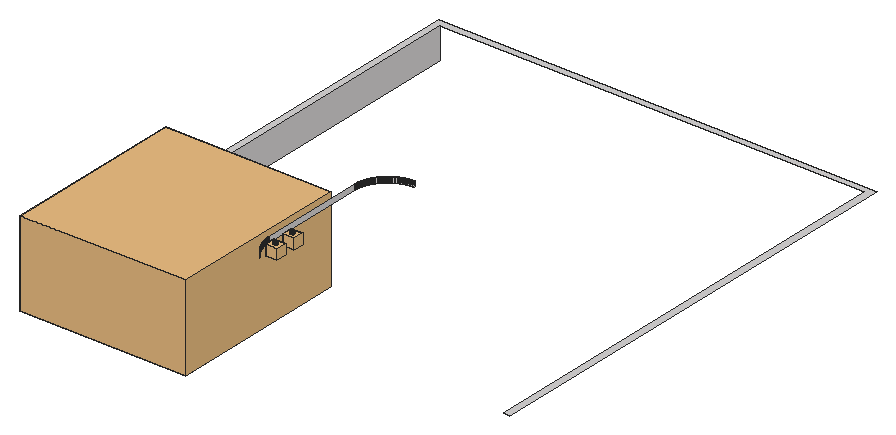
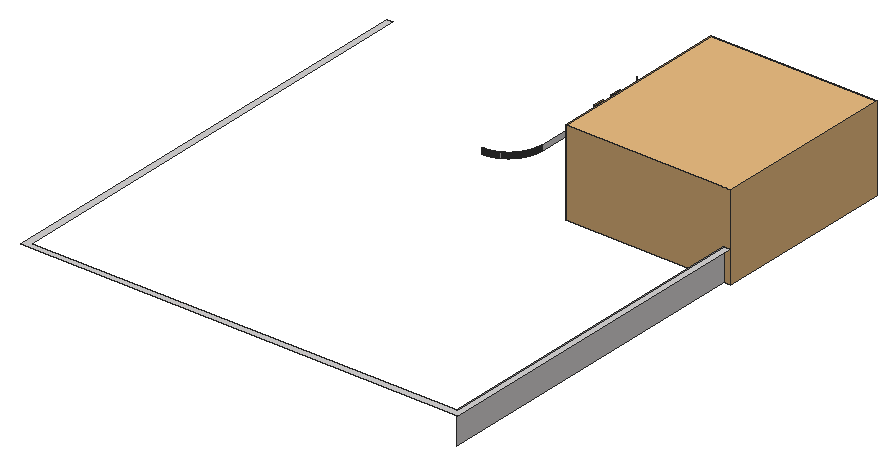
# SketchUp Ruby script. Lengths in inches.
U = 1.inch
M = Sketchup.active_model
def pt(a) = Geom::Point3d.new(a.map { |v| v * U })
def face(e, loops, mat)
  f = e.add_face(loops[0].map { |a| pt(a) })
  loops[1..].each { |l| e.add_face(l.map { |a| pt(a) }).erase! }
  f.material = f.back_material = mat if mat
  f
end
# faces: each face lists its corners as indices into pts; further lists are holes
def faces(e, pts, list, mat = nil) = list.each { |f| face(e, (f[0].is_a?(Array) ? f : [f]).map { |l| l.map { |i| pts[i] } }, mat) }
# xy, xz, yz: faces in a plane at the given z, y or x. An outline is a flat list of corners, or four numbers for a rectangle; further outlines are holes
def ring(l) = l.size == 4 ? [[l[0], l[1]], [l[2], l[1]], [l[2], l[3]], [l[0], l[3]]] : l.each_slice(2).to_a
def flat(e, list, mat, &to3) = list.each { |f| face(e, (f[0].is_a?(Array) ? f : [f]).map { |l| ring(l).map { |u, v| to3.(u, v) } }, mat) }
def xy(e, z, list, mat = nil) = flat(e, list, mat) { |x, y| [x, y, z] }
def xz(e, y, list, mat = nil) = flat(e, list, mat) { |x, z| [x, y, z] }
def yz(e, x, list, mat = nil) = flat(e, list, mat) { |y, z| [x, y, z] }
def lines(e, pts, list) = list.each { |a, b| e.add_line(pt(pts[a]), pt(pts[b])) }
# prism: a flat outline (further loops are holes) pulled along v
def prism(e, loops, v, mat = nil)
  f = face(e, loops, mat); d = Geom::Vector3d.new(v.map { |x| x * U })
  f.pushpull(f.normal.samedirection?(d) ? d.length : -d.length)
end
def box(e, o, s, mat = nil) = prism(e, [[o, [o[0] + s[0], o[1], o[2]], [o[0] + s[0], o[1] + s[1], o[2]], [o[0], o[1] + s[1], o[2]]]], [0, 0, s[2]], mat)
def at(x, y, z, deg = 0) = Geom::Transformation.translation(pt([x, y, z])) * Geom::Transformation.rotation(ORIGIN, Z_AXIS, deg.degrees)
def axes(o, x, y, z) = Geom::Transformation.new([*x, 0, *y, 0, *z, 0, *pt(o).to_a, 1])
def part(name) = M.definitions.add(name)
# library, detail: a bought-in or finely detailed component or shape, given as its bounding box
def library(name, o, s) = part(name).tap { |d| box(d.entities, o, s) }
def detail(e, o, s) = box(e.add_group.entities, o, s)
def put(e, d, t, mat = nil) = e.add_instance(d, t).tap { |i| i.material = mat if mat }
def group(e, t, mat = nil) = e.add_group.tap { |g| g.transformation = t; g.material = mat if mat }.entities
root = M.entities
M.materials.add("[Quartz Light Brown]").color = [215, 212, 212]
M.materials.add("[Wood Veneer 01]").color = [93, 57, 34]
c1 = library("Group\#53",[0,0,-93.56],[180,199,93.56])
c2 = library("3",[-5.26,-4.28,-11.86],[13.52,11.56,11.86])
xy(root,432,[[0,276.5,7,276.5,7,787,488,787,488,276.5,495,276.5,495,794,0,794]],"[Quartz Light Brown]")
xy(root,483,[[193.9375,318.7,193.78,318.71,193.47,318.77,193.32,318.82,193.18,318.88,193.04,318.95,192.9,319.03,192.77,319.12,192.65,319.22,192.54,319.33,192.44,319.45,192.26,319.71,192.19,319.85,192.13,319.99,192.08,320.14,192.04,320.29,192,320.61,192,320.76,192.01,320.92,192.04,321.08,192.07,321.23,192.12,321.38,192.18,321.52,192.25,321.66,192.33,321.8,192.42,321.93,192.52,322.05,192.63,322.16,192.75,322.26,192.875,322.35,193.01,322.4375,193.15,322.51,193.29,322.57,193.44,322.62,193.59,322.66,193.75,322.69,193.91,322.7,194.0625,322.7,194.22,322.6875,194.375,322.67,194.53,322.63,194.68,322.58,194.82,322.52,194.96,322.45,195.1,322.37,195.23,322.28,195.35,322.18,195.46,322.07,195.56,321.95,195.65,321.83,195.74,321.69,195.81,321.55,195.87,321.41,195.92,321.26,195.96,321.11,195.98,320.95,196,320.8,196,320.64,195.99,320.48,195.96,320.33,195.93,320.17,195.88,320.02,195.82,319.88,195.75,319.74,195.67,319.6,195.58,319.48,195.48,319.36,195.37,319.24,195.25,319.14,195.125,319.05,194.99,318.96,194.85,318.89,194.71,318.83,194.56,318.78,194.41,318.74,194.09,318.7],[193.9375,342.7,193.78,342.71,193.47,342.77,193.32,342.82,193.18,342.88,193.04,342.95,192.9,343.03,192.77,343.12,192.65,343.22,192.54,343.33,192.44,343.45,192.26,343.71,192.19,343.85,192.13,343.99,192.08,344.14,192.04,344.29,192,344.61,192,344.76,192.01,344.92,192.04,345.08,192.07,345.23,192.12,345.38,192.18,345.52,192.25,345.66,192.33,345.8,192.42,345.93,192.52,346.05,192.63,346.16,192.75,346.26,192.875,346.35,193.01,346.4375,193.15,346.51,193.29,346.57,193.44,346.62,193.59,346.66,193.75,346.69,193.91,346.7,194.0625,346.7,194.22,346.6875,194.375,346.67,194.53,346.63,194.68,346.58,194.82,346.52,194.96,346.45,195.1,346.37,195.23,346.28,195.35,346.18,195.46,346.07,195.56,345.95,195.65,345.83,195.74,345.69,195.81,345.55,195.87,345.41,195.92,345.26,195.96,345.11,195.98,344.95,196,344.8,196,344.64,195.99,344.48,195.96,344.33,195.93,344.17,195.88,344.02,195.82,343.88,195.75,343.74,195.67,343.6,195.58,343.48,195.48,343.36,195.37,343.24,195.25,343.14,195.125,343.05,194.99,342.96,194.85,342.89,194.71,342.83,194.56,342.78,194.41,342.74,194.09,342.7]],"[Quartz Light Brown]")
xz(root,318.7,[[193.9375,480,194.09,483]],"[Quartz Light Brown]")
xz(root,322.7,[[193.91,480,194.0625,483]],"[Quartz Light Brown]")
xz(root,342.7,[[193.9375,480,194.09,483]],"[Quartz Light Brown]")
xz(root,346.7,[[193.91,480,194.0625,483]],"[Quartz Light Brown]")
xz(root,478.7,[[224.5,480,225,486]],"[Quartz Light Brown]")
yz(root,7,[[276.5,396,787,432]],"[Quartz Light Brown]")
yz(root,187,[[320.2,480,320.7,486],[320.7,480,440.7,486],[440.7,480,441.2,486]],"[Quartz Light Brown]")
yz(root,192,[[320.61,480,320.76,483],[344.61,480,344.76,483]],"[Quartz Light Brown]")
yz(root,196,[[320.64,480,320.8,483],[344.64,480,344.8,483]],"[Quartz Light Brown]")
p = [[198.13,293.83,480],[198.48,293.48,480],[198.48,293.48,486],[198.13,293.83,486],[197.78,294.18,480],[197.78,294.18,486],
  [197.4375,294.54,480],[197.4375,294.54,486],[197.1,294.91,480],[197.1,294.91,486],[196.76,295.27,480],[196.76,295.27,486],
  [196.43,295.65,480],[196.43,295.65,486],[196.1,296.02,480],[196.1,296.02,486],[195.78,296.4,480],[195.78,296.4,486],
  [195.47,296.79,480],[195.47,296.79,486],[195.16,297.18,480],[195.16,297.18,486],[194.85,297.57,480],[194.85,297.57,486],
  [194.55,297.96,480],[194.55,297.96,486],[194.26,298.37,480],[194.26,298.37,486],[193.97,298.77,480],[193.97,298.77,486],
  [193.68,299.18,480],[193.68,299.18,486],[193.4,299.59,480],[193.4,299.59,486],[193.13,300,480],[193.13,300,486],
  [192.86,300.42,480],[192.86,300.42,486],[192.6,300.85,480],[192.6,300.85,486],[192.34,301.27,480],[192.34,301.27,486],
  [192.09,301.7,480],[192.09,301.7,486],[191.85,302.13,480],[191.85,302.13,486],[191.6,302.57,480],[191.6,302.57,486],
  [191.37,303.01,480],[191.37,303.01,486],[191.14,303.45,480],[191.14,303.45,486],[190.92,303.89,480],[190.92,303.89,486],
  [190.7,304.34,480],[190.7,304.34,486],[190.49,304.79,480],[190.49,304.79,486],[190.29,305.25,480],[190.29,305.25,486],
  [190.09,305.7,480],[190.09,305.7,486],[189.89,306.16,480],[189.89,306.16,486],[189.71,306.62,480],[189.71,306.62,486],
  [189.52,307.08,480],[189.52,307.08,486],[189.35,307.55,480],[189.35,307.55,486],[189.18,308.02,480],[189.18,308.02,486],
  [189.02,308.49,480],[189.02,308.49,486],[188.86,308.96,480],[188.86,308.96,486],[188.71,309.43,480],[188.71,309.43,486],
  [188.56,309.91,480],[188.56,309.91,486],[188.43,310.39,480],[188.43,310.39,486],[188.29,310.87,480],[188.29,310.87,486],
  [188.17,311.35,480],[188.17,311.35,486],[188.05,311.83,480],[188.05,311.83,486],[187.9375,312.31,480],[187.9375,312.31,486],
  [187.83,312.8,480],[187.83,312.8,486],[187.73,313.29,480],[187.73,313.29,486],[187.64,313.78,480],[187.64,313.78,486],
  [187.55,314.27,480],[187.55,314.27,486],[187.47,314.76,480],[187.47,314.76,486],[187.39,315.25,480],[187.39,315.25,486],
  [187.33,315.74,480],[187.33,315.74,486],[187.26,316.23,480],[187.26,316.23,486],[187.21,316.73,480],[187.21,316.73,486],
  [187.16,317.22,480],[187.16,317.22,486],[187.12,317.72,480],[187.12,317.72,486],[187.08,318.22,480],[187.08,318.22,486],
  [187.05,318.71,480],[187.05,318.71,486],[187.03,319.21,480],[187.03,319.21,486],[193.625,318.74,480],[193.47,318.77,480],
  [193.47,318.77,483],[193.625,318.74,483],[193.78,318.71,480],[193.78,318.71,483],[193.9375,318.7,480],[193.9375,318.7,483],
  [194.25,318.72,480],[194.09,318.7,480],[194.09,318.7,483],[194.25,318.72,483],[194.41,318.74,480],[194.41,318.74,483],
  [194.56,318.78,480],[194.56,318.78,483],[193.32,318.82,480],[193.18,318.88,480],[193.18,318.88,483],[193.32,318.82,483],
  [194.71,318.83,480],[194.71,318.83,483],[194.85,318.89,480],[194.85,318.89,483],[193.04,318.95,480],[192.9,319.03,480],
  [192.9,319.03,483],[193.04,318.95,483],[194.99,318.96,480],[194.99,318.96,483],[192.77,319.12,480],[192.77,319.12,483],
  [195.125,319.05,480],[195.125,319.05,483],[195.25,319.14,480],[195.25,319.14,483],[192.65,319.22,480],[192.65,319.22,483],
  [195.37,319.24,480],[195.37,319.24,483],[187.01,319.71,480],[187.01,319.71,486],[192.54,319.33,480],[192.54,319.33,483],
  [195.48,319.36,480],[195.48,319.36,483],[192.44,319.45,480],[192.44,319.45,483],[195.58,319.48,480],[195.58,319.48,483],
  [192.35,319.58,480],[192.35,319.58,483],[195.67,319.6,480],[195.67,319.6,483],[192.26,319.71,480],[192.26,319.71,483],
  [195.75,319.74,480],[195.75,319.74,483],[187,320.2,480],[187,320.2,486],[192.19,319.85,480],[192.19,319.85,483],
  [195.82,319.88,480],[195.82,319.88,483],[192.13,319.99,480],[192.13,319.99,483],[195.88,320.02,480],[195.88,320.02,483],
  [192.08,320.14,480],[192.08,320.14,483],[195.93,320.17,480],[195.93,320.17,483],[192.04,320.29,480],[192.04,320.29,483],
  [195.96,320.33,480],[195.96,320.33,483],[192.02,320.45,480],[192.02,320.45,483],[195.99,320.48,480],[195.99,320.48,483],
  [192,320.61,480],[192,320.61,483],[196,320.64,480],[196,320.64,483],[192,320.76,480],[192.01,320.92,480],
  [192.01,320.92,483],[192,320.76,483],[195.98,320.95,480],[196,320.8,480],[196,320.8,483],[195.98,320.95,483],
  [192.04,321.08,480],[192.04,321.08,483],[195.96,321.11,480],[195.96,321.11,483],[192.07,321.23,480],[192.07,321.23,483],
  [195.92,321.26,480],[195.92,321.26,483],[192.12,321.38,480],[192.12,321.38,483],[195.87,321.41,480],[195.87,321.41,483],
  [192.18,321.52,480],[192.18,321.52,483],[195.81,321.55,480],[195.81,321.55,483],[192.25,321.66,480],[192.25,321.66,483],
  [195.74,321.69,480],[195.74,321.69,483],[192.33,321.8,480],[192.33,321.8,483],[195.65,321.83,480],[195.65,321.83,483],
  [192.42,321.93,480],[192.42,321.93,483],[195.56,321.95,480],[195.56,321.95,483],[192.52,322.05,480],[192.52,322.05,483],
  [192.63,322.16,480],[192.63,322.16,483],[195.46,322.07,480],[195.46,322.07,483],[195.35,322.18,480],[195.35,322.18,483],
  [192.75,322.26,480],[192.75,322.26,483],[195.23,322.28,480],[195.23,322.28,483],[192.875,322.35,480],[192.875,322.35,483],
  [195.1,322.37,480],[195.1,322.37,483],[193.01,322.4375,480],[193.01,322.4375,483],[193.15,322.51,480],[193.15,322.51,483],
  [194.96,322.45,480],[194.96,322.45,483],[193.29,322.57,480],[193.29,322.57,483],[194.68,322.58,480],[194.82,322.52,480],
  [194.82,322.52,483],[194.68,322.58,483],[193.44,322.62,480],[193.44,322.62,483],[193.59,322.66,480],[193.59,322.66,483],
  [194.375,322.67,480],[194.53,322.63,480],[194.53,322.63,483],[194.375,322.67,483],[193.75,322.69,480],[193.75,322.69,483],
  [193.91,322.7,480],[193.91,322.7,483],[194.0625,322.7,480],[194.22,322.6875,480],[194.22,322.6875,483],[194.0625,322.7,483],
  [193.625,342.74,480],[193.47,342.77,480],[193.47,342.77,483],[193.625,342.74,483],[193.78,342.71,480],[193.78,342.71,483],
  [193.9375,342.7,480],[193.9375,342.7,483],[194.25,342.72,480],[194.09,342.7,480],[194.09,342.7,483],[194.25,342.72,483],
  [194.41,342.74,480],[194.41,342.74,483],[194.56,342.78,480],[194.56,342.78,483],[193.32,342.82,480],[193.18,342.88,480],
  [193.18,342.88,483],[193.32,342.82,483],[194.71,342.83,480],[194.71,342.83,483],[194.85,342.89,480],[194.85,342.89,483],
  [193.04,342.95,480],[192.9,343.03,480],[192.9,343.03,483],[193.04,342.95,483],[194.99,342.96,480],[194.99,342.96,483],
  [192.77,343.12,480],[192.77,343.12,483],[195.125,343.05,480],[195.125,343.05,483],[195.25,343.14,480],[195.25,343.14,483],
  [192.65,343.22,480],[192.65,343.22,483],[195.37,343.24,480],[195.37,343.24,483],[192.54,343.33,480],[192.54,343.33,483],
  [195.48,343.36,480],[195.48,343.36,483],[192.44,343.45,480],[192.44,343.45,483],[195.58,343.48,480],[195.58,343.48,483],
  [192.35,343.58,480],[192.35,343.58,483],[195.67,343.6,480],[195.67,343.6,483],[192.26,343.71,480],[192.26,343.71,483],
  [195.75,343.74,480],[195.75,343.74,483],[192.19,343.85,480],[192.19,343.85,483],[195.82,343.88,480],[195.82,343.88,483],
  [192.13,343.99,480],[192.13,343.99,483],[195.88,344.02,480],[195.88,344.02,483],[192.08,344.14,480],[192.08,344.14,483],
  [195.93,344.17,480],[195.93,344.17,483],[192.04,344.29,480],[192.04,344.29,483],[195.96,344.33,480],[195.96,344.33,483],
  [192.02,344.45,480],[192.02,344.45,483],[195.99,344.48,480],[195.99,344.48,483],[192,344.61,480],[192,344.61,483],
  [196,344.64,480],[196,344.64,483],[192,344.76,480],[192.01,344.92,480],[192.01,344.92,483],[192,344.76,483],
  [195.98,344.95,480],[196,344.8,480],[196,344.8,483],[195.98,344.95,483],[192.04,345.08,480],[192.04,345.08,483],
  [195.96,345.11,480],[195.96,345.11,483],[192.07,345.23,480],[192.07,345.23,483],[195.92,345.26,480],[195.92,345.26,483],
  [192.12,345.38,480],[192.12,345.38,483],[195.87,345.41,480],[195.87,345.41,483],[192.18,345.52,480],[192.18,345.52,483],
  [195.81,345.55,480],[195.81,345.55,483],[192.25,345.66,480],[192.25,345.66,483],[195.74,345.69,480],[195.74,345.69,483],
  [192.33,345.8,480],[192.33,345.8,483],[195.65,345.83,480],[195.65,345.83,483],[192.42,345.93,480],[192.42,345.93,483],
  [195.56,345.95,480],[195.56,345.95,483],[192.52,346.05,480],[192.52,346.05,483],[192.63,346.16,480],[192.63,346.16,483],
  [195.46,346.07,480],[195.46,346.07,483],[195.35,346.18,480],[195.35,346.18,483],[192.75,346.26,480],[192.75,346.26,483],
  [195.23,346.28,480],[195.23,346.28,483],[192.875,346.35,480],[192.875,346.35,483],[195.1,346.37,480],[195.1,346.37,483],
  [193.01,346.4375,480],[193.01,346.4375,483],[193.15,346.51,480],[193.15,346.51,483],[194.96,346.45,480],[194.96,346.45,483],
  [193.29,346.57,480],[193.29,346.57,483],[194.68,346.58,480],[194.82,346.52,480],[194.82,346.52,483],[194.68,346.58,483],
  [193.44,346.62,480],[193.44,346.62,483],[193.59,346.66,480],[193.59,346.66,483],[194.375,346.67,480],[194.53,346.63,480],
  [194.53,346.63,483],[194.375,346.67,483],[193.75,346.69,480],[193.75,346.69,483],[193.91,346.7,480],[193.91,346.7,483],
  [194.0625,346.7,480],[194.22,346.6875,480],[194.22,346.6875,483],[194.0625,346.7,483],[187.01,441.7,480],[187,441.2,480],
  [187,441.2,486],[187.01,441.7,486],[187.03,442.19,480],[187.03,442.19,486],[187.05,442.69,480],[187.05,442.69,486],
  [187.08,443.1875,480],[187.08,443.1875,486],[187.12,443.68,480],[187.12,443.68,486],[187.16,444.18,480],[187.16,444.18,486],
  [187.21,444.67,480],[187.21,444.67,486],[187.26,445.17,480],[187.26,445.17,486],[187.33,445.66,480],[187.33,445.66,486],
  [187.39,446.15,480],[187.39,446.15,486],[187.47,446.65,480],[187.47,446.65,486],[187.55,447.14,480],[187.55,447.14,486],
  [187.64,447.625,480],[187.64,447.625,486],[187.73,448.11,480],[187.73,448.11,486],[187.83,448.6,480],[187.83,448.6,486],
  [187.9375,449.09,480],[187.9375,449.09,486],[188.05,449.57,480],[188.05,449.57,486],[188.17,450.05,480],[188.17,450.05,486],
  [188.29,450.54,480],[188.29,450.54,486],[188.43,451.02,480],[188.43,451.02,486],[188.56,451.49,480],[188.56,451.49,486],
  [188.71,451.97,480],[188.71,451.97,486],[188.86,452.44,480],[188.86,452.44,486],[189.02,452.92,480],[189.02,452.92,486],
  [189.18,453.39,480],[189.18,453.39,486],[189.35,453.85,480],[189.35,453.85,486],[189.52,454.32,480],[189.52,454.32,486],
  [189.71,454.78,480],[189.71,454.78,486],[189.89,455.24,480],[189.89,455.24,486],[190.09,455.7,480],[190.09,455.7,486],
  [190.29,456.16,480],[190.29,456.16,486],[190.49,456.61,480],[190.49,456.61,486],[190.7,457.06,480],[190.7,457.06,486],
  [190.92,457.51,480],[190.92,457.51,486],[191.14,457.95,480],[191.14,457.95,486],[191.37,458.39,480],[191.37,458.39,486],
  [191.6,458.83,480],[191.6,458.83,486],[191.85,459.27,480],[191.85,459.27,486],[192.09,459.7,480],[192.09,459.7,486],
  [192.34,460.13,480],[192.34,460.13,486],[192.6,460.56,480],[192.6,460.56,486],[192.86,460.98,480],[192.86,460.98,486],
  [193.13,461.4,480],[193.13,461.4,486],[193.4,461.8125,480],[193.4,461.8125,486],[193.68,462.22,480],[193.68,462.22,486],
  [193.97,462.63,480],[193.97,462.63,486],[194.26,463.04,480],[194.26,463.04,486],[194.55,463.4375,480],[194.55,463.4375,486],
  [194.85,463.83,480],[194.85,463.83,486],[195.16,464.23,480],[195.16,464.23,486],[195.47,464.62,480],[195.47,464.62,486],
  [195.78,465,480],[195.78,465,486],[196.1,465.38,480],[196.1,465.38,486],[196.43,465.76,480],[196.43,465.76,486],
  [196.76,466.13,480],[196.76,466.13,486],[197.1,466.5,480],[197.1,466.5,486],[197.4375,466.86,480],[197.4375,466.86,486],
  [197.78,467.22,480],[197.78,467.22,486],[198.13,467.57,480],[198.13,467.57,486],[198.48,467.92,480],[198.48,467.92,486],
  [198.84,468.27,480],[198.84,468.27,486],[199.21,468.61,480],[199.21,468.61,486],[199.57,468.94,480],[199.57,468.94,486],
  [199.94,469.27,480],[199.94,469.27,486],[200.32,469.6,480],[200.32,469.6,486],[200.7,469.92,480],[200.7,469.92,486],
  [201.09,470.23,480],[201.09,470.23,486],[201.47,470.54,480],[201.47,470.54,486],[201.87,470.85,480],[201.87,470.85,486],
  [202.26,471.15,480],[202.26,471.15,486],[202.66,471.44,480],[202.66,471.44,486],[203.07,471.73,480],[203.07,471.73,486],
  [203.48,472.02,480],[203.48,472.02,486],[203.89,472.3,480],[203.89,472.3,486],[204.3,472.57,480],[204.3,472.57,486],
  [204.72,472.84,480],[204.72,472.84,486],[205.15,473.1,480],[205.15,473.1,486],[205.57,473.36,480],[205.57,473.36,486],
  [206,473.61,480],[206,473.61,486],[206.43,473.86,480],[206.43,473.86,486],[206.87,474.1,480],[206.87,474.1,486],
  [207.31,474.33,480],[207.31,474.33,486],[207.75,474.56,480],[207.75,474.56,486],[208.19,474.78,480],[208.19,474.78,486],
  [208.64,475,480],[208.64,475,486],[209.09,475.21,480],[209.09,475.21,486],[209.54,475.42,480],[209.54,475.42,486],
  [210,475.62,480],[210,475.62,486],[210.46,475.81,480],[210.46,475.81,486],[210.92,476,480],[210.92,476,486],
  [211.38,476.18,480],[211.38,476.18,486],[211.85,476.35,480],[211.85,476.35,486],[212.32,476.52,480],[212.32,476.52,486],
  [212.79,476.68,480],[212.79,476.68,486],[213.26,476.84,480],[213.26,476.84,486],[213.73,476.99,480],[213.73,476.99,486],
  [214.21,477.14,480],[214.21,477.14,486],[214.69,477.27,480],[214.69,477.27,486],[215.16,477.41,480],[215.16,477.41,486],
  [215.65,477.53,480],[215.65,477.53,486],[216.13,477.65,480],[216.13,477.65,486],[216.61,477.76,480],[216.61,477.76,486],
  [217.1,477.87,480],[217.1,477.87,486],[217.59,477.97,480],[217.59,477.97,486],[218.08,478.06,480],[218.08,478.06,486],
  [218.56,478.15,480],[218.56,478.15,486],[219.06,478.23,480],[219.06,478.23,486],[219.55,478.31,480],[219.55,478.31,486],
  [220.04,478.375,480],[220.04,478.375,486],[220.53,478.4375,480],[220.53,478.4375,486],[221.03,478.49,480],[221.03,478.49,486],
  [221.52,478.54,480],[221.52,478.54,486],[222.02,478.58,480],[222.02,478.58,486],[222.51,478.62,480],[222.51,478.62,486],
  [223.01,478.65,480],[223.01,478.65,486],[223.51,478.67,480],[223.51,478.67,486],[224.01,478.6875,480],[224.01,478.6875,486],
  [224.5,478.7,480],[224.5,478.7,486]]
faces(root,p,[[0,1,2,3],[4,0,3,5],[6,4,5,7],[8,6,7,9],[10,8,9,11],[12,10,11,13],[14,12,13,15],[16,14,15,17],
  [18,16,17,19],[20,18,19,21],[22,20,21,23],[24,22,23,25],[26,24,25,27],[28,26,27,29],[30,28,29,31],[32,30,31,33],
  [34,32,33,35],[36,34,35,37],[38,36,37,39],[40,38,39,41],[42,40,41,43],[44,42,43,45],[46,44,45,47],[48,46,47,49],
  [50,48,49,51],[52,50,51,53],[54,52,53,55],[56,54,55,57],[58,56,57,59],[60,58,59,61],[62,60,61,63],[64,62,63,65],
  [66,64,65,67],[68,66,67,69],[70,68,69,71],[72,70,71,73],[74,72,73,75],[76,74,75,77],[78,76,77,79],[80,78,79,81],
  [82,80,81,83],[84,82,83,85],[86,84,85,87],[88,86,87,89],[90,88,89,91],[92,90,91,93],[94,92,93,95],[96,94,95,97],
  [98,96,97,99],[100,98,99,101],[102,100,101,103],[104,102,103,105],[106,104,105,107],[108,106,107,109],[110,108,109,111],[112,110,111,113],
  [114,112,113,115],[116,114,115,117],[118,119,120,121],[122,118,121,123],[124,122,123,125],[126,127,128,129],[130,126,129,131],[132,130,131,133],
  [134,135,136,137],[119,134,137,120],[138,132,133,139],[140,138,139,141],[142,143,144,145],[135,142,145,136],[146,140,141,147],[143,148,149,144],
  [150,146,147,151],[152,150,151,153],[148,154,155,149],[156,152,153,157],[158,116,117,159],[154,160,161,155],[162,156,157,163],[160,164,165,161],
  [166,162,163,167],[164,168,169,165],[170,166,167,171],[168,172,173,169],[174,170,171,175],[176,158,159,177],[172,178,179,173],[180,174,175,181],
  [178,182,183,179],[184,180,181,185],[182,186,187,183],[188,184,185,189],[186,190,191,187],[192,188,189,193],[190,194,195,191],[196,192,193,197],
  [194,198,199,195],[200,196,197,201],[202,203,204,205],[206,207,208,209],[203,210,211,204],[212,206,209,213],[210,214,215,211],[216,212,213,217],
  [214,218,219,215],[220,216,217,221],[218,222,223,219],[224,220,221,225],[222,226,227,223],[228,224,225,229],[226,230,231,227],[232,228,229,233],
  [230,234,235,231],[236,232,233,237],[234,238,239,235],[238,240,241,239],[242,236,237,243],[244,242,243,245],[240,246,247,241],[248,244,245,249],
  [246,250,251,247],[252,248,249,253],[250,254,255,251],[254,256,257,255],[258,252,253,259],[256,260,261,257],[262,263,264,265],[263,258,259,264],
  [260,266,267,261],[266,268,269,267],[270,271,272,273],[271,262,265,272],[268,274,275,269],[274,276,277,275],[278,279,280,281],[279,270,273,280],
  [282,283,284,285],[286,282,285,287],[288,286,287,289],[290,291,292,293],[294,290,293,295],[296,294,295,297],[298,299,300,301],[283,298,301,284],
  [302,296,297,303],[304,302,303,305],[306,307,308,309],[299,306,309,300],[310,304,305,311],[307,312,313,308],[314,310,311,315],[316,314,315,317],
  [312,318,319,313],[320,316,317,321],[318,322,323,319],[324,320,321,325],[322,326,327,323],[328,324,325,329],[326,330,331,327],[332,328,329,333],
  [330,334,335,331],[336,332,333,337],[334,338,339,335],[340,336,337,341],[338,342,343,339],[344,340,341,345],[342,346,347,343],[348,344,345,349],
  [346,350,351,347],[352,348,349,353],[350,354,355,351],[356,352,353,357],[354,358,359,355],[360,356,357,361],[362,363,364,365],[366,367,368,369],
  [363,370,371,364],[372,366,369,373],[370,374,375,371],[376,372,373,377],[374,378,379,375],[380,376,377,381],[378,382,383,379],[384,380,381,385],
  [382,386,387,383],[388,384,385,389],[386,390,391,387],[392,388,389,393],[390,394,395,391],[396,392,393,397],[394,398,399,395],[398,400,401,399],
  [402,396,397,403],[404,402,403,405],[400,406,407,401],[408,404,405,409],[406,410,411,407],[412,408,409,413],[410,414,415,411],[414,416,417,415],
  [418,412,413,419],[416,420,421,417],[422,423,424,425],[423,418,419,424],[420,426,427,421],[426,428,429,427],[430,431,432,433],[431,422,425,432],
  [428,434,435,429],[434,436,437,435],[438,439,440,441],[439,430,433,440],[442,443,444,445],[446,442,445,447],[448,446,447,449],[450,448,449,451],
  [452,450,451,453],[454,452,453,455],[456,454,455,457],[458,456,457,459],[460,458,459,461],[462,460,461,463],[464,462,463,465],[466,464,465,467],
  [468,466,467,469],[470,468,469,471],[472,470,471,473],[474,472,473,475],[476,474,475,477],[478,476,477,479],[480,478,479,481],[482,480,481,483],
  [484,482,483,485],[486,484,485,487],[488,486,487,489],[490,488,489,491],[492,490,491,493],[494,492,493,495],[496,494,495,497],[498,496,497,499],
  [500,498,499,501],[502,500,501,503],[504,502,503,505],[506,504,505,507],[508,506,507,509],[510,508,509,511],[512,510,511,513],[514,512,513,515],
  [516,514,515,517],[518,516,517,519],[520,518,519,521],[522,520,521,523],[524,522,523,525],[526,524,525,527],[528,526,527,529],[530,528,529,531],
  [532,530,531,533],[534,532,533,535],[536,534,535,537],[538,536,537,539],[540,538,539,541],[542,540,541,543],[544,542,543,545],[546,544,545,547],
  [548,546,547,549],[550,548,549,551],[552,550,551,553],[554,552,553,555],[556,554,555,557],[558,556,557,559],[560,558,559,561],[562,560,561,563],
  [564,562,563,565],[566,564,565,567],[568,566,567,569],[570,568,569,571],[572,570,571,573],[574,572,573,575],[576,574,575,577],[578,576,577,579],
  [580,578,579,581],[582,580,581,583],[584,582,583,585],[586,584,585,587],[588,586,587,589],[590,588,589,591],[592,590,591,593],[594,592,593,595],
  [596,594,595,597],[598,596,597,599],[600,598,599,601],[602,600,601,603],[604,602,603,605],[606,604,605,607],[608,606,607,609],[610,608,609,611],
  [612,610,611,613],[614,612,613,615],[616,614,615,617],[618,616,617,619],[620,618,619,621],[622,620,621,623],[624,622,623,625],[626,624,625,627],
  [628,626,627,629],[630,628,629,631],[632,630,631,633],[634,632,633,635],[636,634,635,637],[638,636,637,639],[640,638,639,641],[642,640,641,643],
  [644,642,643,645],[646,644,645,647],[648,646,647,649],[650,648,649,651],[652,650,651,653],[654,652,653,655],[656,654,655,657],[658,656,657,659],
  [660,658,659,661],[662,660,661,663],[664,662,663,665],[666,664,665,667],[668,666,667,669],[670,668,669,671],[672,670,671,673],[674,672,673,675],
  [676,674,675,677],[678,676,677,679]],"[Quartz Light Brown]")
put(root,c1,axes([-1.1875,204.03,492.37],[1.03803,0,0],[0,1.03103,0],[0,0,1.03]),"[Wood Veneer 01]")
put(root,c2,at(192.5,319.2,481.25),"[Quartz Light Brown]")
put(root,c2,at(192.5,343.2,481.25),"[Quartz Light Brown]")
